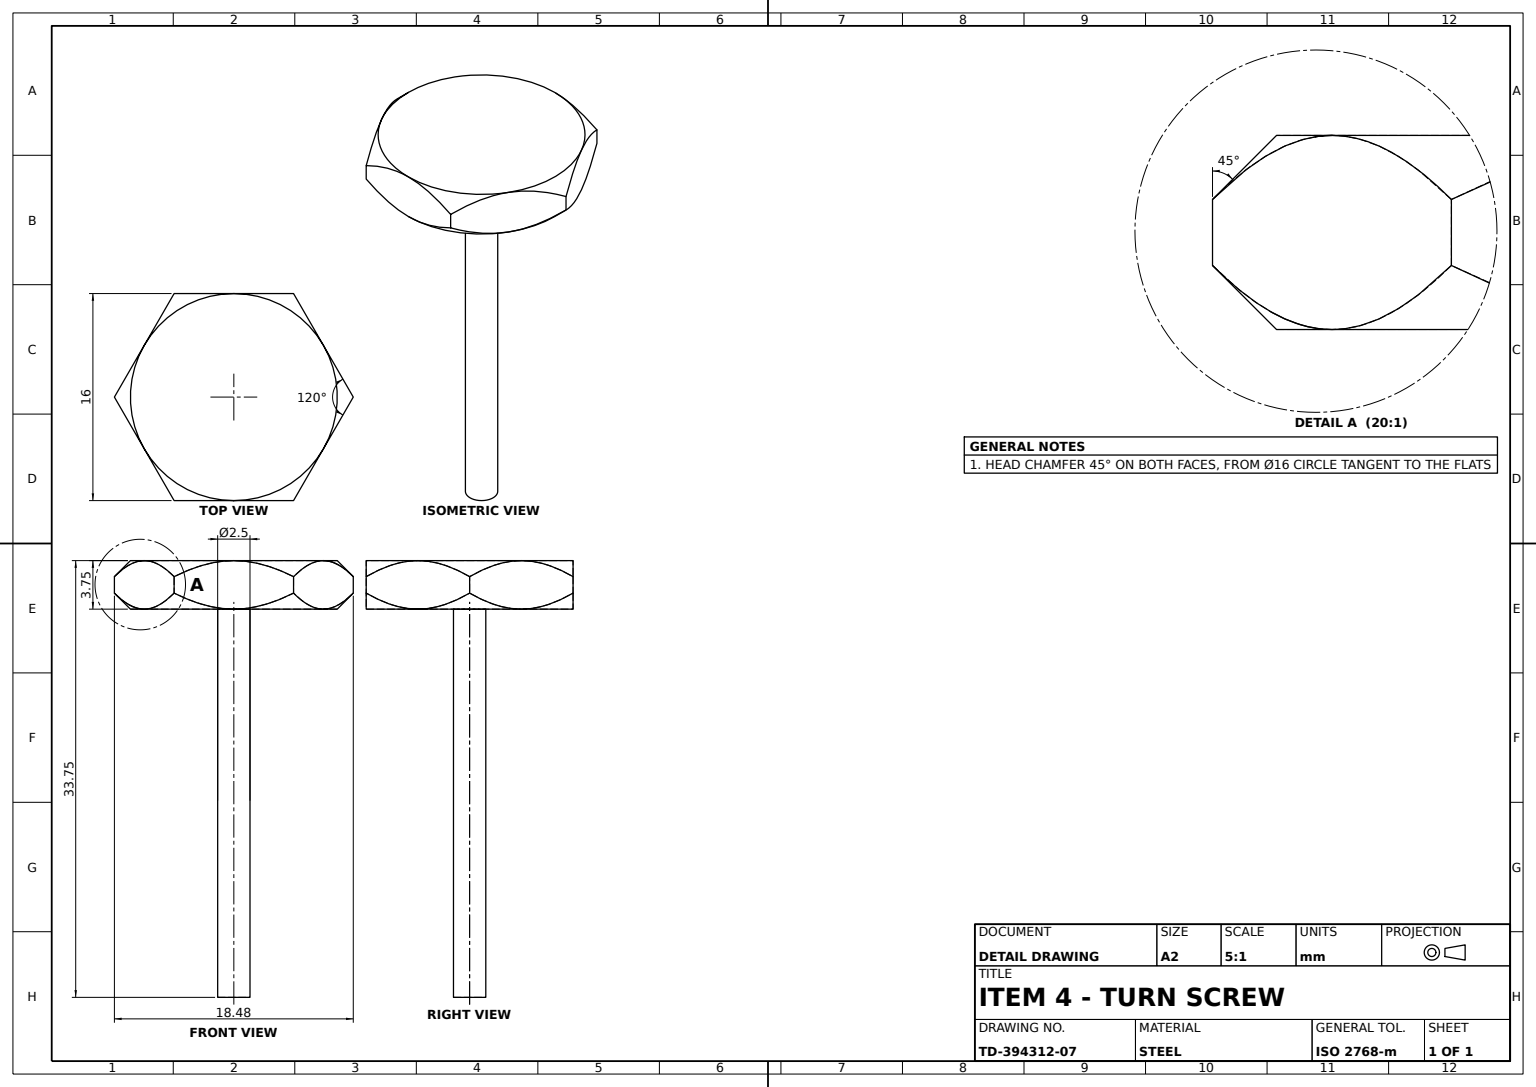
ISO-10303-21;
HEADER;
FILE_DESCRIPTION((''),'2;1');
FILE_NAME('','',(''),(''),'','','');
FILE_SCHEMA(('AUTOMOTIVE_DESIGN'));
ENDSEC;
DATA;
#1=APPLICATION_CONTEXT('');
#2=PRODUCT_CONTEXT('',#1,'mechanical');
#3=PRODUCT('','','',(#2));
#4=PRODUCT_DEFINITION_FORMATION('','',#3);
#5=PRODUCT_DEFINITION_CONTEXT('',#1,'design');
#6=PRODUCT_DEFINITION('','',#4,#5);
#7=PRODUCT_DEFINITION_SHAPE('','',#6);
#8=(LENGTH_UNIT()NAMED_UNIT(*)SI_UNIT(.MILLI.,.METRE.));
#9=(NAMED_UNIT(*)PLANE_ANGLE_UNIT()SI_UNIT($,.RADIAN.));
#10=(NAMED_UNIT(*)SI_UNIT($,.STERADIAN.)SOLID_ANGLE_UNIT());
#11=UNCERTAINTY_MEASURE_WITH_UNIT(LENGTH_MEASURE(1.E-05),#8,'distance_accuracy_value','');
#12=(GEOMETRIC_REPRESENTATION_CONTEXT(3)GLOBAL_UNCERTAINTY_ASSIGNED_CONTEXT((#11))GLOBAL_UNIT_ASSIGNED_CONTEXT((#8,#9,#10))REPRESENTATION_CONTEXT('',''));
#13=CARTESIAN_POINT('',(0.,3.75,8.));
#14=VERTEX_POINT('',#13);
#15=CARTESIAN_POINT('',(4.618802,2.512396,8.));
#16=VERTEX_POINT('',#15);
#17=CARTESIAN_POINT('',(0.406471,3.75,8.));
#18=CARTESIAN_POINT('',(0.810745,3.718564,8.));
#19=CARTESIAN_POINT('',(1.602792,3.600424,8.));
#20=CARTESIAN_POINT('',(1.992753,3.513803,8.));
#21=CARTESIAN_POINT('',(3.147431,3.184847,8.));
#22=CARTESIAN_POINT('',(3.901866,2.870864,8.));
#23=B_SPLINE_CURVE_WITH_KNOTS('',3,(#13,#17,#18,#19,#20,#21,#22,#15),.UNSPECIFIED.,.F.,.F.,(4,2,2,4),(0.017278831,0.018482156,0.01968548,0.022092129),.UNSPECIFIED.);
#24=EDGE_CURVE('',#14,#16,#23,.T.);
#25=ORIENTED_EDGE('',*,*,#24,.T.);
#26=CARTESIAN_POINT('',(6.928203,3.75,4.));
#27=VERTEX_POINT('',#26);
#28=CARTESIAN_POINT('',(4.980949,2.874543,7.372743));
#29=CARTESIAN_POINT('',(5.351293,3.182274,6.731289));
#30=CARTESIAN_POINT('',(5.926776,3.511295,5.734523));
#31=CARTESIAN_POINT('',(6.121967,3.598638,5.396441));
#32=CARTESIAN_POINT('',(6.520646,3.718248,4.70591));
#33=CARTESIAN_POINT('',(6.725938,3.75,4.350334));
#34=B_SPLINE_CURVE_WITH_KNOTS('',3,(#15,#28,#29,#30,#31,#32,#33,#26),.UNSPECIFIED.,.F.,.F.,(4,2,2,4),(0.000000254,0.002394158,0.00359111,0.004788061),.UNSPECIFIED.);
#35=EDGE_CURVE('',#16,#27,#34,.T.);
#36=ORIENTED_EDGE('',*,*,#35,.T.);
#37=CARTESIAN_POINT('',(0.,3.75,0.));
#38=DIRECTION('',(0.,1.,0.));
#39=DIRECTION('',(0.,0.,1.));
#40=AXIS2_PLACEMENT_3D('',#37,#38,#39);
#41=CIRCLE('',#40,8.);
#42=EDGE_CURVE('',#14,#27,#41,.T.);
#43=ORIENTED_EDGE('',*,*,#42,.F.);
#44=EDGE_LOOP('',(#25,#36,#43));
#45=FACE_OUTER_BOUND('',#44,.T.);
#46=DIRECTION('',(0.,-1.,0.));
#47=AXIS2_PLACEMENT_3D('',#37,#46,#39);
#48=CONICAL_SURFACE('',#47,8.,0.785398163);
#49=ADVANCED_FACE('',(#45),#48,.T.);
#50=CARTESIAN_POINT('',(-9.237604,2.512396,0.));
#51=VERTEX_POINT('',#50);
#52=CARTESIAN_POINT('',(-6.928203,3.75,4.));
#53=VERTEX_POINT('',#52);
#54=CARTESIAN_POINT('',(-8.875457,2.874543,0.627257));
#55=CARTESIAN_POINT('',(-8.505114,3.182274,1.268711));
#56=CARTESIAN_POINT('',(-7.92963,3.511295,2.265477));
#57=CARTESIAN_POINT('',(-7.734439,3.598638,2.603559));
#58=CARTESIAN_POINT('',(-7.335761,3.718248,3.29409));
#59=CARTESIAN_POINT('',(-7.130469,3.75,3.649666));
#60=B_SPLINE_CURVE_WITH_KNOTS('',3,(#50,#54,#55,#56,#57,#58,#59,#52),.UNSPECIFIED.,.F.,.F.,(4,2,2,4),(0.000000254,0.002394158,0.00359111,0.004788061),.UNSPECIFIED.);
#61=EDGE_CURVE('',#51,#53,#60,.T.);
#62=ORIENTED_EDGE('',*,*,#61,.T.);
#63=CARTESIAN_POINT('',(-6.928203,3.75,-4.));
#64=VERTEX_POINT('',#63);
#65=EDGE_CURVE('',#64,#53,#41,.T.);
#66=ORIENTED_EDGE('',*,*,#65,.F.);
#67=CARTESIAN_POINT('',(-7.329901,3.75,-3.30424));
#68=CARTESIAN_POINT('',(-7.724768,3.627157,-2.62031));
#69=CARTESIAN_POINT('',(-8.503545,3.184411,-1.271428));
#70=CARTESIAN_POINT('',(-8.875876,2.874124,-0.626531));
#71=B_SPLINE_CURVE_WITH_KNOTS('',3,(#63,#67,#68,#69,#70,#50),.UNSPECIFIED.,.F.,.F.,(4,2,4),(0.004788061,0.007165196,0.009542331),.UNSPECIFIED.);
#72=EDGE_CURVE('',#64,#51,#71,.T.);
#73=ORIENTED_EDGE('',*,*,#72,.T.);
#74=EDGE_LOOP('',(#62,#66,#73));
#75=FACE_OUTER_BOUND('',#74,.T.);
#76=ADVANCED_FACE('',(#75),#48,.T.);
#77=ORIENTED_EDGE('',*,*,#65,.T.);
#78=EDGE_CURVE('',#53,#14,#41,.T.);
#79=ORIENTED_EDGE('',*,*,#78,.T.);
#80=ORIENTED_EDGE('',*,*,#42,.T.);
#81=CARTESIAN_POINT('',(6.928203,3.75,-4.));
#82=VERTEX_POINT('',#81);
#83=EDGE_CURVE('',#27,#82,#41,.T.);
#84=ORIENTED_EDGE('',*,*,#83,.T.);
#85=CARTESIAN_POINT('',(0.,3.75,-8.));
#86=VERTEX_POINT('',#85);
#87=EDGE_CURVE('',#82,#86,#41,.T.);
#88=ORIENTED_EDGE('',*,*,#87,.T.);
#89=EDGE_CURVE('',#86,#64,#41,.T.);
#90=ORIENTED_EDGE('',*,*,#89,.T.);
#91=EDGE_LOOP('',(#77,#79,#80,#84,#88,#90));
#92=FACE_OUTER_BOUND('',#91,.T.);
#93=PLANE('',#40);
#94=ADVANCED_FACE('',(#92),#93,.T.);
#95=CARTESIAN_POINT('',(9.237604,2.512396,0.));
#96=VERTEX_POINT('',#95);
#97=CARTESIAN_POINT('',(9.237604,1.237604,0.));
#98=VERTEX_POINT('',#97);
#99=CARTESIAN_POINT('',(9.237604,3.75,0.));
#100=VECTOR('',#46,1000.);
#101=LINE('',#99,#100);
#102=EDGE_CURVE('',#96,#98,#101,.T.);
#103=ORIENTED_EDGE('',*,*,#102,.F.);
#104=CARTESIAN_POINT('',(7.329901,3.75,3.30424));
#105=CARTESIAN_POINT('',(7.724768,3.627157,2.62031));
#106=CARTESIAN_POINT('',(8.503545,3.184411,1.271428));
#107=CARTESIAN_POINT('',(8.875876,2.874124,0.626531));
#108=B_SPLINE_CURVE_WITH_KNOTS('',3,(#26,#104,#105,#106,#107,#95),.UNSPECIFIED.,.F.,.F.,(4,2,4),(0.004788061,0.007165196,0.009542331),.UNSPECIFIED.);
#109=EDGE_CURVE('',#27,#96,#108,.T.);
#110=ORIENTED_EDGE('',*,*,#109,.F.);
#111=ORIENTED_EDGE('',*,*,#35,.F.);
#112=CARTESIAN_POINT('',(4.618802,1.237604,8.));
#113=VERTEX_POINT('',#112);
#114=CARTESIAN_POINT('',(4.618802,3.75,8.));
#115=LINE('',#114,#100);
#116=EDGE_CURVE('',#16,#113,#115,.T.);
#117=ORIENTED_EDGE('',*,*,#116,.T.);
#118=CARTESIAN_POINT('',(6.928203,0.,4.));
#119=VERTEX_POINT('',#118);
#120=CARTESIAN_POINT('',(6.526506,0.,4.69576));
#121=CARTESIAN_POINT('',(6.131639,0.122843,5.37969));
#122=CARTESIAN_POINT('',(5.352862,0.565589,6.728572));
#123=CARTESIAN_POINT('',(4.98053,0.875876,7.373469));
#124=B_SPLINE_CURVE_WITH_KNOTS('',3,(#118,#120,#121,#122,#123,#112),.UNSPECIFIED.,.F.,.F.,(4,2,4),(0.004788061,0.007165196,0.009542331),.UNSPECIFIED.);
#125=EDGE_CURVE('',#119,#113,#124,.T.);
#126=ORIENTED_EDGE('',*,*,#125,.F.);
#127=CARTESIAN_POINT('',(8.875457,0.875457,0.627257));
#128=CARTESIAN_POINT('',(8.505114,0.567726,1.268711));
#129=CARTESIAN_POINT('',(7.92963,0.238705,2.265477));
#130=CARTESIAN_POINT('',(7.734439,0.151362,2.603559));
#131=CARTESIAN_POINT('',(7.335761,0.031752,3.29409));
#132=CARTESIAN_POINT('',(7.130469,0.,3.649666));
#133=B_SPLINE_CURVE_WITH_KNOTS('',3,(#97,#127,#128,#129,#130,#131,#132,#118),.UNSPECIFIED.,.F.,.F.,(4,2,2,4),(0.000000254,0.002394158,0.00359111,0.004788061),.UNSPECIFIED.);
#134=EDGE_CURVE('',#98,#119,#133,.T.);
#135=ORIENTED_EDGE('',*,*,#134,.F.);
#136=EDGE_LOOP('',(#103,#110,#111,#117,#126,#135));
#137=FACE_OUTER_BOUND('',#136,.T.);
#138=DIRECTION('',(-0.866025404,0.,-0.5));
#139=DIRECTION('',(-0.5,0.,0.866025404));
#140=AXIS2_PLACEMENT_3D('',#114,#138,#139);
#141=PLANE('',#140);
#142=ADVANCED_FACE('',(#137),#141,.F.);
#143=CARTESIAN_POINT('',(0.,-30.,1.25));
#144=VERTEX_POINT('',#143);
#145=CARTESIAN_POINT('',(0.,-30.,-1.25));
#146=VERTEX_POINT('',#145);
#147=CARTESIAN_POINT('',(0.,-30.,0.));
#148=DIRECTION('',(0.,0.,-1.));
#149=AXIS2_PLACEMENT_3D('',#147,#46,#148);
#150=CIRCLE('',#149,1.25);
#151=EDGE_CURVE('',#144,#146,#150,.T.);
#152=ORIENTED_EDGE('',*,*,#151,.T.);
#153=EDGE_CURVE('',#146,#144,#150,.T.);
#154=ORIENTED_EDGE('',*,*,#153,.T.);
#155=EDGE_LOOP('',(#152,#154));
#156=FACE_OUTER_BOUND('',#155,.T.);
#157=PLANE('',#149);
#158=ADVANCED_FACE('',(#156),#157,.T.);
#159=CARTESIAN_POINT('',(6.928203,0.,-4.));
#160=VERTEX_POINT('',#159);
#161=CARTESIAN_POINT('',(7.329901,0.,-3.30424));
#162=CARTESIAN_POINT('',(7.724768,0.122843,-2.62031));
#163=CARTESIAN_POINT('',(8.503545,0.565589,-1.271428));
#164=CARTESIAN_POINT('',(8.875876,0.875876,-0.626531));
#165=B_SPLINE_CURVE_WITH_KNOTS('',3,(#159,#161,#162,#163,#164,#97),.UNSPECIFIED.,.F.,.F.,(4,2,4),(0.004788061,0.007165196,0.009542331),.UNSPECIFIED.);
#166=EDGE_CURVE('',#160,#98,#165,.T.);
#167=ORIENTED_EDGE('',*,*,#166,.T.);
#168=ORIENTED_EDGE('',*,*,#134,.T.);
#169=CARTESIAN_POINT('',(0.,0.,0.));
#170=AXIS2_PLACEMENT_3D('',#169,#38,#39);
#171=CIRCLE('',#170,8.);
#172=EDGE_CURVE('',#119,#160,#171,.T.);
#173=ORIENTED_EDGE('',*,*,#172,.T.);
#174=EDGE_LOOP('',(#167,#168,#173));
#175=FACE_OUTER_BOUND('',#174,.T.);
#176=AXIS2_PLACEMENT_3D('',#169,#38,#148);
#177=CONICAL_SURFACE('',#176,8.,0.785398163);
#178=ADVANCED_FACE('',(#175),#177,.T.);
#179=ORIENTED_EDGE('',*,*,#116,.F.);
#180=ORIENTED_EDGE('',*,*,#24,.F.);
#181=CARTESIAN_POINT('',(-4.618802,2.512396,8.));
#182=VERTEX_POINT('',#181);
#183=CARTESIAN_POINT('',(-4.260257,2.691668,8.));
#184=CARTESIAN_POINT('',(-3.894538,2.859032,8.));
#185=CARTESIAN_POINT('',(-3.143604,3.161396,8.));
#186=CARTESIAN_POINT('',(-2.760704,3.295136,8.));
#187=CARTESIAN_POINT('',(-1.603396,3.624496,8.));
#188=CARTESIAN_POINT('',(-0.813767,3.75,8.));
#189=B_SPLINE_CURVE_WITH_KNOTS('',3,(#181,#183,#184,#185,#186,#187,#188,#13),.UNSPECIFIED.,.F.,.F.,(4,2,2,4),(0.012460655,0.013665199,0.014869743,0.017278831),.UNSPECIFIED.);
#190=EDGE_CURVE('',#182,#14,#189,.T.);
#191=ORIENTED_EDGE('',*,*,#190,.F.);
#192=CARTESIAN_POINT('',(-4.618802,1.237604,8.));
#193=VERTEX_POINT('',#192);
#194=CARTESIAN_POINT('',(-4.618802,3.75,8.));
#195=LINE('',#194,#100);
#196=EDGE_CURVE('',#182,#193,#195,.T.);
#197=ORIENTED_EDGE('',*,*,#196,.T.);
#198=CARTESIAN_POINT('',(0.,0.,8.));
#199=VERTEX_POINT('',#198);
#200=CARTESIAN_POINT('',(-0.406471,0.,8.));
#201=CARTESIAN_POINT('',(-0.810745,0.031436,8.));
#202=CARTESIAN_POINT('',(-1.602792,0.149576,8.));
#203=CARTESIAN_POINT('',(-1.992753,0.236197,8.));
#204=CARTESIAN_POINT('',(-3.147431,0.565153,8.));
#205=CARTESIAN_POINT('',(-3.901866,0.879136,8.));
#206=B_SPLINE_CURVE_WITH_KNOTS('',3,(#198,#200,#201,#202,#203,#204,#205,#192),.UNSPECIFIED.,.F.,.F.,(4,2,2,4),(0.017278831,0.018482156,0.01968548,0.022092129),.UNSPECIFIED.);
#207=EDGE_CURVE('',#199,#193,#206,.T.);
#208=ORIENTED_EDGE('',*,*,#207,.F.);
#209=CARTESIAN_POINT('',(4.260257,1.058332,8.));
#210=CARTESIAN_POINT('',(3.894538,0.890968,8.));
#211=CARTESIAN_POINT('',(3.143604,0.588604,8.));
#212=CARTESIAN_POINT('',(2.760704,0.454864,8.));
#213=CARTESIAN_POINT('',(1.603396,0.125504,8.));
#214=CARTESIAN_POINT('',(0.813767,0.,8.));
#215=B_SPLINE_CURVE_WITH_KNOTS('',3,(#112,#209,#210,#211,#212,#213,#214,#198),.UNSPECIFIED.,.F.,.F.,(4,2,2,4),(0.012460655,0.013665199,0.014869743,0.017278831),.UNSPECIFIED.);
#216=EDGE_CURVE('',#113,#199,#215,.T.);
#217=ORIENTED_EDGE('',*,*,#216,.F.);
#218=EDGE_LOOP('',(#179,#180,#191,#197,#208,#217));
#219=FACE_OUTER_BOUND('',#218,.T.);
#220=DIRECTION('',(-1.,0.,0.));
#221=AXIS2_PLACEMENT_3D('',#194,#148,#220);
#222=PLANE('',#221);
#223=ADVANCED_FACE('',(#219),#222,.F.);
#224=CARTESIAN_POINT('',(0.,0.,-8.));
#225=VERTEX_POINT('',#224);
#226=CARTESIAN_POINT('',(4.618802,1.237604,-8.));
#227=VERTEX_POINT('',#226);
#228=CARTESIAN_POINT('',(0.406471,0.,-8.));
#229=CARTESIAN_POINT('',(0.810745,0.031436,-8.));
#230=CARTESIAN_POINT('',(1.602792,0.149576,-8.));
#231=CARTESIAN_POINT('',(1.992753,0.236197,-8.));
#232=CARTESIAN_POINT('',(3.147431,0.565153,-8.));
#233=CARTESIAN_POINT('',(3.901866,0.879136,-8.));
#234=B_SPLINE_CURVE_WITH_KNOTS('',3,(#224,#228,#229,#230,#231,#232,#233,#226),.UNSPECIFIED.,.F.,.F.,(4,2,2,4),(0.017278831,0.018482156,0.01968548,0.022092129),.UNSPECIFIED.);
#235=EDGE_CURVE('',#225,#227,#234,.T.);
#236=ORIENTED_EDGE('',*,*,#235,.T.);
#237=CARTESIAN_POINT('',(4.980949,0.875457,-7.372743));
#238=CARTESIAN_POINT('',(5.351293,0.567726,-6.731289));
#239=CARTESIAN_POINT('',(5.926776,0.238705,-5.734523));
#240=CARTESIAN_POINT('',(6.121967,0.151362,-5.396441));
#241=CARTESIAN_POINT('',(6.520646,0.031752,-4.70591));
#242=CARTESIAN_POINT('',(6.725938,0.,-4.350334));
#243=B_SPLINE_CURVE_WITH_KNOTS('',3,(#226,#237,#238,#239,#240,#241,#242,#159),.UNSPECIFIED.,.F.,.F.,(4,2,2,4),(0.000000254,0.002394158,0.00359111,0.004788061),.UNSPECIFIED.);
#244=EDGE_CURVE('',#227,#160,#243,.T.);
#245=ORIENTED_EDGE('',*,*,#244,.T.);
#246=AXIS2_PLACEMENT_3D('',#169,#46,#148);
#247=CIRCLE('',#246,8.);
#248=EDGE_CURVE('',#225,#160,#247,.T.);
#249=ORIENTED_EDGE('',*,*,#248,.F.);
#250=EDGE_LOOP('',(#236,#245,#249));
#251=FACE_OUTER_BOUND('',#250,.T.);
#252=ADVANCED_FACE('',(#251),#177,.T.);
#253=ORIENTED_EDGE('',*,*,#235,.F.);
#254=CARTESIAN_POINT('',(-4.618802,1.237604,-8.));
#255=VERTEX_POINT('',#254);
#256=CARTESIAN_POINT('',(-4.260257,1.058332,-8.));
#257=CARTESIAN_POINT('',(-3.894538,0.890968,-8.));
#258=CARTESIAN_POINT('',(-3.143604,0.588604,-8.));
#259=CARTESIAN_POINT('',(-2.760704,0.454864,-8.));
#260=CARTESIAN_POINT('',(-1.603396,0.125504,-8.));
#261=CARTESIAN_POINT('',(-0.813767,0.,-8.));
#262=B_SPLINE_CURVE_WITH_KNOTS('',3,(#254,#256,#257,#258,#259,#260,#261,#224),.UNSPECIFIED.,.F.,.F.,(4,2,2,4),(0.012460655,0.013665199,0.014869743,0.017278831),.UNSPECIFIED.);
#263=EDGE_CURVE('',#255,#225,#262,.T.);
#264=ORIENTED_EDGE('',*,*,#263,.F.);
#265=CARTESIAN_POINT('',(-4.618802,2.512396,-8.));
#266=VERTEX_POINT('',#265);
#267=CARTESIAN_POINT('',(-4.618802,3.75,-8.));
#268=LINE('',#267,#100);
#269=EDGE_CURVE('',#266,#255,#268,.T.);
#270=ORIENTED_EDGE('',*,*,#269,.F.);
#271=CARTESIAN_POINT('',(-0.406471,3.75,-8.));
#272=CARTESIAN_POINT('',(-0.810745,3.718564,-8.));
#273=CARTESIAN_POINT('',(-1.602792,3.600424,-8.));
#274=CARTESIAN_POINT('',(-1.992753,3.513803,-8.));
#275=CARTESIAN_POINT('',(-3.147431,3.184847,-8.));
#276=CARTESIAN_POINT('',(-3.901866,2.870864,-8.));
#277=B_SPLINE_CURVE_WITH_KNOTS('',3,(#85,#271,#272,#273,#274,#275,#276,#265),.UNSPECIFIED.,.F.,.F.,(4,2,2,4),(0.017278831,0.018482156,0.01968548,0.022092129),.UNSPECIFIED.);
#278=EDGE_CURVE('',#86,#266,#277,.T.);
#279=ORIENTED_EDGE('',*,*,#278,.F.);
#280=CARTESIAN_POINT('',(4.618802,2.512396,-8.));
#281=VERTEX_POINT('',#280);
#282=CARTESIAN_POINT('',(4.260257,2.691668,-8.));
#283=CARTESIAN_POINT('',(3.894538,2.859032,-8.));
#284=CARTESIAN_POINT('',(3.143604,3.161396,-8.));
#285=CARTESIAN_POINT('',(2.760704,3.295136,-8.));
#286=CARTESIAN_POINT('',(1.603396,3.624496,-8.));
#287=CARTESIAN_POINT('',(0.813767,3.75,-8.));
#288=B_SPLINE_CURVE_WITH_KNOTS('',3,(#280,#282,#283,#284,#285,#286,#287,#85),.UNSPECIFIED.,.F.,.F.,(4,2,2,4),(0.012460655,0.013665199,0.014869743,0.017278831),.UNSPECIFIED.);
#289=EDGE_CURVE('',#281,#86,#288,.T.);
#290=ORIENTED_EDGE('',*,*,#289,.F.);
#291=CARTESIAN_POINT('',(4.618802,3.75,-8.));
#292=LINE('',#291,#100);
#293=EDGE_CURVE('',#281,#227,#292,.T.);
#294=ORIENTED_EDGE('',*,*,#293,.T.);
#295=EDGE_LOOP('',(#253,#264,#270,#279,#290,#294));
#296=FACE_OUTER_BOUND('',#295,.T.);
#297=DIRECTION('',(1.,0.,0.));
#298=AXIS2_PLACEMENT_3D('',#291,#39,#297);
#299=PLANE('',#298);
#300=ADVANCED_FACE('',(#296),#299,.F.);
#301=CARTESIAN_POINT('',(-6.526506,3.75,4.69576));
#302=CARTESIAN_POINT('',(-6.131639,3.627157,5.37969));
#303=CARTESIAN_POINT('',(-5.352862,3.184411,6.728572));
#304=CARTESIAN_POINT('',(-4.98053,2.874124,7.373469));
#305=B_SPLINE_CURVE_WITH_KNOTS('',3,(#52,#301,#302,#303,#304,#181),.UNSPECIFIED.,.F.,.F.,(4,2,4),(0.004788061,0.007165196,0.009542331),.UNSPECIFIED.);
#306=EDGE_CURVE('',#53,#182,#305,.T.);
#307=ORIENTED_EDGE('',*,*,#306,.T.);
#308=ORIENTED_EDGE('',*,*,#190,.T.);
#309=ORIENTED_EDGE('',*,*,#78,.F.);
#310=EDGE_LOOP('',(#307,#308,#309));
#311=FACE_OUTER_BOUND('',#310,.T.);
#312=ADVANCED_FACE('',(#311),#48,.T.);
#313=ORIENTED_EDGE('',*,*,#153,.F.);
#314=CARTESIAN_POINT('',(0.,0.,-1.25));
#315=VERTEX_POINT('',#314);
#316=VECTOR('',#38,1000.);
#317=LINE('',#145,#316);
#318=EDGE_CURVE('',#146,#315,#317,.T.);
#319=ORIENTED_EDGE('',*,*,#318,.T.);
#320=CARTESIAN_POINT('',(0.,0.,1.25));
#321=VERTEX_POINT('',#320);
#322=AXIS2_PLACEMENT_3D('',#169,#46,#39);
#323=CIRCLE('',#322,1.25);
#324=EDGE_CURVE('',#315,#321,#323,.T.);
#325=ORIENTED_EDGE('',*,*,#324,.T.);
#326=LINE('',#143,#316);
#327=EDGE_CURVE('',#144,#321,#326,.T.);
#328=ORIENTED_EDGE('',*,*,#327,.F.);
#329=EDGE_LOOP('',(#313,#319,#325,#328));
#330=FACE_OUTER_BOUND('',#329,.T.);
#331=AXIS2_PLACEMENT_3D('',#147,#38,#39);
#332=CYLINDRICAL_SURFACE('',#331,1.25);
#333=ADVANCED_FACE('',(#330),#332,.T.);
#334=CARTESIAN_POINT('',(-9.237604,1.237604,0.));
#335=VERTEX_POINT('',#334);
#336=CARTESIAN_POINT('',(-6.928203,0.,-4.));
#337=VERTEX_POINT('',#336);
#338=CARTESIAN_POINT('',(-8.875457,0.875457,-0.627257));
#339=CARTESIAN_POINT('',(-8.505114,0.567726,-1.268711));
#340=CARTESIAN_POINT('',(-7.92963,0.238705,-2.265477));
#341=CARTESIAN_POINT('',(-7.734439,0.151362,-2.603559));
#342=CARTESIAN_POINT('',(-7.335761,0.031752,-3.29409));
#343=CARTESIAN_POINT('',(-7.130469,0.,-3.649666));
#344=B_SPLINE_CURVE_WITH_KNOTS('',3,(#334,#338,#339,#340,#341,#342,#343,#336),.UNSPECIFIED.,.F.,.F.,(4,2,2,4),(0.000000254,0.002394158,0.00359111,0.004788061),.UNSPECIFIED.);
#345=EDGE_CURVE('',#335,#337,#344,.T.);
#346=ORIENTED_EDGE('',*,*,#345,.T.);
#347=CARTESIAN_POINT('',(-6.928203,0.,4.));
#348=VERTEX_POINT('',#347);
#349=EDGE_CURVE('',#337,#348,#171,.T.);
#350=ORIENTED_EDGE('',*,*,#349,.T.);
#351=CARTESIAN_POINT('',(-7.329901,0.,3.30424));
#352=CARTESIAN_POINT('',(-7.724768,0.122843,2.62031));
#353=CARTESIAN_POINT('',(-8.503545,0.565589,1.271428));
#354=CARTESIAN_POINT('',(-8.875876,0.875876,0.626531));
#355=B_SPLINE_CURVE_WITH_KNOTS('',3,(#347,#351,#352,#353,#354,#334),.UNSPECIFIED.,.F.,.F.,(4,2,4),(0.004788061,0.007165196,0.009542331),.UNSPECIFIED.);
#356=EDGE_CURVE('',#348,#335,#355,.T.);
#357=ORIENTED_EDGE('',*,*,#356,.T.);
#358=EDGE_LOOP('',(#346,#350,#357));
#359=FACE_OUTER_BOUND('',#358,.T.);
#360=ADVANCED_FACE('',(#359),#177,.T.);
#361=CARTESIAN_POINT('',(8.875457,2.874543,-0.627257));
#362=CARTESIAN_POINT('',(8.505114,3.182274,-1.268711));
#363=CARTESIAN_POINT('',(7.92963,3.511295,-2.265477));
#364=CARTESIAN_POINT('',(7.734439,3.598638,-2.603559));
#365=CARTESIAN_POINT('',(7.335761,3.718248,-3.29409));
#366=CARTESIAN_POINT('',(7.130469,3.75,-3.649666));
#367=B_SPLINE_CURVE_WITH_KNOTS('',3,(#95,#361,#362,#363,#364,#365,#366,#81),.UNSPECIFIED.,.F.,.F.,(4,2,2,4),(0.000000254,0.002394158,0.00359111,0.004788061),.UNSPECIFIED.);
#368=EDGE_CURVE('',#96,#82,#367,.T.);
#369=ORIENTED_EDGE('',*,*,#368,.T.);
#370=ORIENTED_EDGE('',*,*,#83,.F.);
#371=ORIENTED_EDGE('',*,*,#109,.T.);
#372=EDGE_LOOP('',(#369,#370,#371));
#373=FACE_OUTER_BOUND('',#372,.T.);
#374=ADVANCED_FACE('',(#373),#48,.T.);
#375=ORIENTED_EDGE('',*,*,#324,.F.);
#376=EDGE_CURVE('',#321,#315,#323,.T.);
#377=ORIENTED_EDGE('',*,*,#376,.F.);
#378=EDGE_LOOP('',(#375,#377));
#379=FACE_BOUND('',#378,.T.);
#380=ORIENTED_EDGE('',*,*,#172,.F.);
#381=EDGE_CURVE('',#199,#119,#171,.T.);
#382=ORIENTED_EDGE('',*,*,#381,.F.);
#383=EDGE_CURVE('',#348,#199,#171,.T.);
#384=ORIENTED_EDGE('',*,*,#383,.F.);
#385=ORIENTED_EDGE('',*,*,#349,.F.);
#386=EDGE_CURVE('',#225,#337,#171,.T.);
#387=ORIENTED_EDGE('',*,*,#386,.F.);
#388=ORIENTED_EDGE('',*,*,#248,.T.);
#389=EDGE_LOOP('',(#380,#382,#384,#385,#387,#388));
#390=FACE_OUTER_BOUND('',#389,.T.);
#391=PLANE('',#170);
#392=ADVANCED_FACE('',(#379,#390),#391,.F.);
#393=ORIENTED_EDGE('',*,*,#151,.F.);
#394=ORIENTED_EDGE('',*,*,#327,.T.);
#395=ORIENTED_EDGE('',*,*,#376,.T.);
#396=ORIENTED_EDGE('',*,*,#318,.F.);
#397=EDGE_LOOP('',(#393,#394,#395,#396));
#398=FACE_OUTER_BOUND('',#397,.T.);
#399=ADVANCED_FACE('',(#398),#332,.T.);
#400=ORIENTED_EDGE('',*,*,#125,.T.);
#401=ORIENTED_EDGE('',*,*,#216,.T.);
#402=ORIENTED_EDGE('',*,*,#381,.T.);
#403=EDGE_LOOP('',(#400,#401,#402));
#404=FACE_OUTER_BOUND('',#403,.T.);
#405=ADVANCED_FACE('',(#404),#177,.T.);
#406=ORIENTED_EDGE('',*,*,#383,.T.);
#407=ORIENTED_EDGE('',*,*,#207,.T.);
#408=CARTESIAN_POINT('',(-4.980949,0.875457,7.372743));
#409=CARTESIAN_POINT('',(-5.351293,0.567726,6.731289));
#410=CARTESIAN_POINT('',(-5.926776,0.238705,5.734523));
#411=CARTESIAN_POINT('',(-6.121967,0.151362,5.396441));
#412=CARTESIAN_POINT('',(-6.520646,0.031752,4.70591));
#413=CARTESIAN_POINT('',(-6.725938,0.,4.350334));
#414=B_SPLINE_CURVE_WITH_KNOTS('',3,(#192,#408,#409,#410,#411,#412,#413,#347),.UNSPECIFIED.,.F.,.F.,(4,2,2,4),(0.000000254,0.002394158,0.00359111,0.004788061),.UNSPECIFIED.);
#415=EDGE_CURVE('',#193,#348,#414,.T.);
#416=ORIENTED_EDGE('',*,*,#415,.T.);
#417=EDGE_LOOP('',(#406,#407,#416));
#418=FACE_OUTER_BOUND('',#417,.T.);
#419=ADVANCED_FACE('',(#418),#177,.T.);
#420=CARTESIAN_POINT('',(-9.237604,3.75,0.));
#421=LINE('',#420,#100);
#422=EDGE_CURVE('',#51,#335,#421,.T.);
#423=ORIENTED_EDGE('',*,*,#422,.T.);
#424=ORIENTED_EDGE('',*,*,#356,.F.);
#425=ORIENTED_EDGE('',*,*,#415,.F.);
#426=ORIENTED_EDGE('',*,*,#196,.F.);
#427=ORIENTED_EDGE('',*,*,#306,.F.);
#428=ORIENTED_EDGE('',*,*,#61,.F.);
#429=EDGE_LOOP('',(#423,#424,#425,#426,#427,#428));
#430=FACE_OUTER_BOUND('',#429,.T.);
#431=DIRECTION('',(0.866025404,0.,-0.5));
#432=DIRECTION('',(-0.5,0.,-0.866025404));
#433=AXIS2_PLACEMENT_3D('',#420,#431,#432);
#434=PLANE('',#433);
#435=ADVANCED_FACE('',(#430),#434,.F.);
#436=CARTESIAN_POINT('',(-4.980949,2.874543,-7.372743));
#437=CARTESIAN_POINT('',(-5.351293,3.182274,-6.731289));
#438=CARTESIAN_POINT('',(-5.926776,3.511295,-5.734523));
#439=CARTESIAN_POINT('',(-6.121967,3.598638,-5.396441));
#440=CARTESIAN_POINT('',(-6.520646,3.718248,-4.70591));
#441=CARTESIAN_POINT('',(-6.725938,3.75,-4.350334));
#442=B_SPLINE_CURVE_WITH_KNOTS('',3,(#265,#436,#437,#438,#439,#440,#441,#63),.UNSPECIFIED.,.F.,.F.,(4,2,2,4),(0.000000254,0.002394158,0.00359111,0.004788061),.UNSPECIFIED.);
#443=EDGE_CURVE('',#266,#64,#442,.T.);
#444=ORIENTED_EDGE('',*,*,#443,.T.);
#445=ORIENTED_EDGE('',*,*,#89,.F.);
#446=ORIENTED_EDGE('',*,*,#278,.T.);
#447=EDGE_LOOP('',(#444,#445,#446));
#448=FACE_OUTER_BOUND('',#447,.T.);
#449=ADVANCED_FACE('',(#448),#48,.T.);
#450=ORIENTED_EDGE('',*,*,#244,.F.);
#451=ORIENTED_EDGE('',*,*,#293,.F.);
#452=CARTESIAN_POINT('',(6.526506,3.75,-4.69576));
#453=CARTESIAN_POINT('',(6.131639,3.627157,-5.37969));
#454=CARTESIAN_POINT('',(5.352862,3.184411,-6.728572));
#455=CARTESIAN_POINT('',(4.98053,2.874124,-7.373469));
#456=B_SPLINE_CURVE_WITH_KNOTS('',3,(#81,#452,#453,#454,#455,#280),.UNSPECIFIED.,.F.,.F.,(4,2,4),(0.004788061,0.007165196,0.009542331),.UNSPECIFIED.);
#457=EDGE_CURVE('',#82,#281,#456,.T.);
#458=ORIENTED_EDGE('',*,*,#457,.F.);
#459=ORIENTED_EDGE('',*,*,#368,.F.);
#460=ORIENTED_EDGE('',*,*,#102,.T.);
#461=ORIENTED_EDGE('',*,*,#166,.F.);
#462=EDGE_LOOP('',(#450,#451,#458,#459,#460,#461));
#463=FACE_OUTER_BOUND('',#462,.T.);
#464=DIRECTION('',(-0.866025404,0.,0.5));
#465=DIRECTION('',(0.5,0.,0.866025404));
#466=AXIS2_PLACEMENT_3D('',#99,#464,#465);
#467=PLANE('',#466);
#468=ADVANCED_FACE('',(#463),#467,.F.);
#469=ORIENTED_EDGE('',*,*,#289,.T.);
#470=ORIENTED_EDGE('',*,*,#87,.F.);
#471=ORIENTED_EDGE('',*,*,#457,.T.);
#472=EDGE_LOOP('',(#469,#470,#471));
#473=FACE_OUTER_BOUND('',#472,.T.);
#474=ADVANCED_FACE('',(#473),#48,.T.);
#475=ORIENTED_EDGE('',*,*,#422,.F.);
#476=ORIENTED_EDGE('',*,*,#72,.F.);
#477=ORIENTED_EDGE('',*,*,#443,.F.);
#478=ORIENTED_EDGE('',*,*,#269,.T.);
#479=CARTESIAN_POINT('',(-6.526506,0.,-4.69576));
#480=CARTESIAN_POINT('',(-6.131639,0.122843,-5.37969));
#481=CARTESIAN_POINT('',(-5.352862,0.565589,-6.728572));
#482=CARTESIAN_POINT('',(-4.98053,0.875876,-7.373469));
#483=B_SPLINE_CURVE_WITH_KNOTS('',3,(#336,#479,#480,#481,#482,#254),.UNSPECIFIED.,.F.,.F.,(4,2,4),(0.004788061,0.007165196,0.009542331),.UNSPECIFIED.);
#484=EDGE_CURVE('',#337,#255,#483,.T.);
#485=ORIENTED_EDGE('',*,*,#484,.F.);
#486=ORIENTED_EDGE('',*,*,#345,.F.);
#487=EDGE_LOOP('',(#475,#476,#477,#478,#485,#486));
#488=FACE_OUTER_BOUND('',#487,.T.);
#489=DIRECTION('',(0.866025404,0.,0.5));
#490=DIRECTION('',(0.5,0.,-0.866025404));
#491=AXIS2_PLACEMENT_3D('',#267,#489,#490);
#492=PLANE('',#491);
#493=ADVANCED_FACE('',(#488),#492,.F.);
#494=ORIENTED_EDGE('',*,*,#386,.T.);
#495=ORIENTED_EDGE('',*,*,#484,.T.);
#496=ORIENTED_EDGE('',*,*,#263,.T.);
#497=EDGE_LOOP('',(#494,#495,#496));
#498=FACE_OUTER_BOUND('',#497,.T.);
#499=ADVANCED_FACE('',(#498),#177,.T.);
#500=CLOSED_SHELL('',(#49,#76,#94,#142,#158,#178,#223,#252,#300,#312,#333,#360,#374,#392,#399,#405,#419,#435,#449,#468,#474,#493,#499));
#501=MANIFOLD_SOLID_BREP('',#500);
#502=ADVANCED_BREP_SHAPE_REPRESENTATION('',(#501),#12);
#503=SHAPE_DEFINITION_REPRESENTATION(#7,#502);
ENDSEC;
END-ISO-10303-21;
